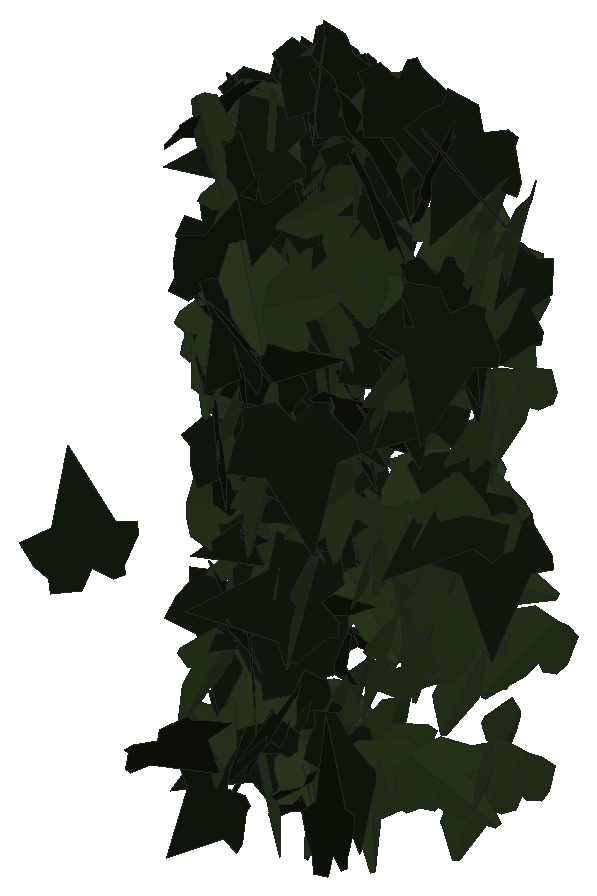
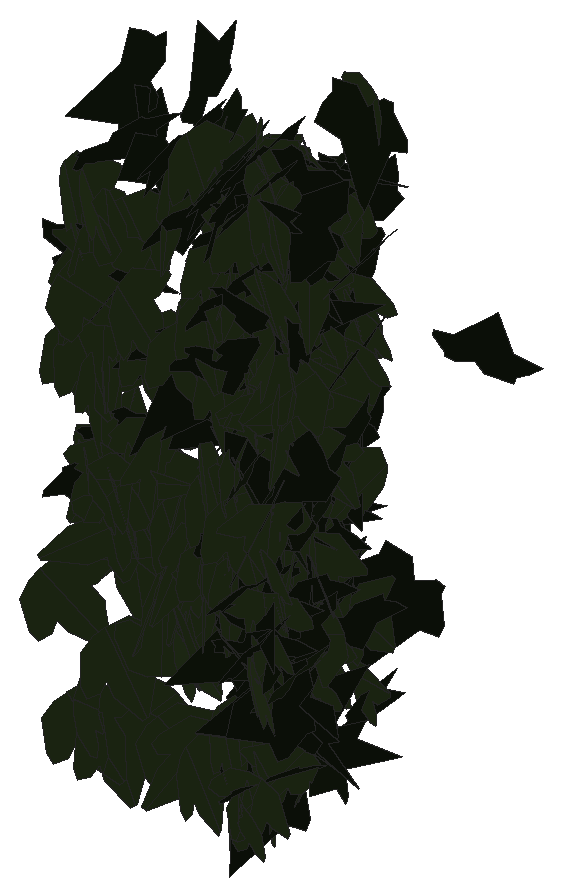
# SketchUp Ruby script. Lengths in inches.
U = 1.inch
M = Sketchup.active_model
def pt(a) = Geom::Point3d.new(a.map { |v| v * U })
def face(e, loops, mat)
  f = e.add_face(loops[0].map { |a| pt(a) })
  loops[1..].each { |l| e.add_face(l.map { |a| pt(a) }).erase! }
  f.material = f.back_material = mat if mat
  f
end
# faces: each face lists its corners as indices into pts; further lists are holes
def faces(e, pts, list, mat = nil) = list.each { |f| face(e, (f[0].is_a?(Array) ? f : [f]).map { |l| l.map { |i| pts[i] } }, mat) }
# xy, xz, yz: faces in a plane at the given z, y or x. An outline is a flat list of corners, or four numbers for a rectangle; further outlines are holes
def ring(l) = l.size == 4 ? [[l[0], l[1]], [l[2], l[1]], [l[2], l[3]], [l[0], l[3]]] : l.each_slice(2).to_a
def flat(e, list, mat, &to3) = list.each { |f| face(e, (f[0].is_a?(Array) ? f : [f]).map { |l| ring(l).map { |u, v| to3.(u, v) } }, mat) }
def xy(e, z, list, mat = nil) = flat(e, list, mat) { |x, y| [x, y, z] }
def xz(e, y, list, mat = nil) = flat(e, list, mat) { |x, z| [x, y, z] }
def yz(e, x, list, mat = nil) = flat(e, list, mat) { |y, z| [x, y, z] }
def lines(e, pts, list) = list.each { |a, b| e.add_line(pt(pts[a]), pt(pts[b])) }
# prism: a flat outline (further loops are holes) pulled along v
def prism(e, loops, v, mat = nil)
  f = face(e, loops, mat); d = Geom::Vector3d.new(v.map { |x| x * U })
  f.pushpull(f.normal.samedirection?(d) ? d.length : -d.length)
end
def box(e, o, s, mat = nil) = prism(e, [[o, [o[0] + s[0], o[1], o[2]], [o[0] + s[0], o[1] + s[1], o[2]], [o[0], o[1] + s[1], o[2]]]], [0, 0, s[2]], mat)
def at(x, y, z, deg = 0) = Geom::Transformation.translation(pt([x, y, z])) * Geom::Transformation.rotation(ORIGIN, Z_AXIS, deg.degrees)
def axes(o, x, y, z) = Geom::Transformation.new([*x, 0, *y, 0, *z, 0, *pt(o).to_a, 1])
def part(name) = M.definitions.add(name)
# library, detail: a bought-in or finely detailed component or shape, given as its bounding box
def library(name, o, s) = part(name).tap { |d| box(d.entities, o, s) }
def detail(e, o, s) = box(e.add_group.entities, o, s)
def put(e, d, t, mat = nil) = e.add_instance(d, t).tap { |i| i.material = mat if mat }
def group(e, t, mat = nil) = e.add_group.tap { |g| g.transformation = t; g.material = mat if mat }.entities
root = M.entities
M.materials.add("efeu1").color = [18, 25, 13]
M.materials.add("efeu2").color = [43, 57, 29]
c1 = part("ivyleaf_9")
p = [[1.54,2.16,1.25],[1.36,2.04,1.19],[-0.21,0.99,0.68],[-0.71,1.11,0.82],[-0.85,0.86,0.67],[-0.8,0.17,0.21],
  [-0.9,-0.01,0.1],[-0.67,-0.16,-0.02],[-0.08,-0.08,-0.05],[-0.03,-0.6,-0.4],[0.65,-0.88,-0.66],[0.83,-0.6,-0.49],
  [1.29,-0.42,-0.43],[1.8125,-0.07,-0.26],[1.21,0.44,0.15]]
faces(c1.entities,p,[[0,1,2,3,4,5,6,7,8,9,10,11,12,13,14]],"efeu1")
c2 = part("ivyleaf_10")
p = [[0,0.5,-0.03],[-0.0625,2.02,-0.43],[-0.19,2.01,-0.46],[-0.54,1.05,-0.29],[-0.52,0.625,-0.18],[-0.83,0.76,-0.28],
  [-1.16,0.64,-0.33],[-1.15,0.33,-0.24],[-0.77,-0.39,0.02],[-0.3,-0.51,0.16],[0.04,-0.48,0.23],[-0.02,2.01,-0.4375],
  [-0.06,2.01,-0.43],[0.04,-0.49,0.23],[0.67,-0.49,0.14],[1.38,0.36,-0.2],[1.375,0.51,-0.24],[0.81,0.65,-0.19],
  [0.62,0.59,-0.15],[0.6,1.09,-0.28],[0.5,1.23,-0.31]]
faces(c2.entities,p,[[0,1,2,3,4,5,6,7,8,9,10],[11,12,0,13,14,15,16,17,18,19,20]],"efeu2")
put(root,c1,axes([9.03,220.3,218.375],[-0.46158,-0.0625,0.05363],[0.05614,0.00087,0.44916],[-0.06712,0.43049,0.00688]))
put(root,c1,axes([9.21,221.32,215.71],[0.26243,0.35078,0.08782],[0.05444,0.0678,-0.44379],[-0.38585,0.24815,-0.00288]))
put(root,c1,axes([10.73,221.81,220.03],[-0.17094,-0.39097,-0.26062],[0.10894,0.2368,-0.42668],[0.45707,-0.20266,0.00422]))
put(root,c2,axes([10.66,222.125,217.94],[0.22138,-0.35038,0.27968],[0.16796,-0.22438,-0.41405],[0.41567,0.27728,0.01836]))
put(root,c1,axes([9.42,222.5,220.57],[-0.01869,-0.3188,0.38473],[-0.022,-0.3841,-0.31935],[0.49917,-0.02886,0.00033]))
put(root,c1,axes([9.09,222.61,214.48],[-0.1098,-0.3044,0.30539],[-0.09865,-0.27908,-0.33376],[0.44601,-0.13666,0.00136]))
put(root,c1,axes([9.27,222.56,219.99],[0.00235,-0.06151,0.4962],[0.13344,-0.47813,-0.0599],[0.48186,0.1327,0.01417]))
put(root,c1,axes([9.27,222.16,220.86],[0.45081,-0.04213,-0.11954],[-0.12069,0.03558,-0.43565],[0.05398,0.43149,0.02425]))
put(root,c1,axes([9.29,222.26,219.22],[0.12737,-0.03029,-0.43432],[-0.44087,0.0882,-0.12654],[0.1006,0.42489,-0.0047]))
put(root,c1,axes([9.15,222.26,221.14],[-0.10416,-0.16282,0.40735],[0.33014,0.2518,0.18714],[-0.3176,0.31514,0.06094]))
put(root,c2,axes([8.84,222.77,216.06],[0.00663,-0.31537,0.31153],[0.07081,-0.29549,-0.32493],[0.46439,0.04956,0.0451]))
put(root,c1,axes([10.82,222.36,214.46],[-0.06273,-0.27844,0.41053],[0.07774,0.40317,0.28533],[-0.48992,0.09963,-0.00729]))
put(root,c2,axes([9.42,222.51,221.33],[0.44175,0.16313,0.16806],[0.15784,0.05773,-0.47091],[-0.17304,0.4691,-0.00049]))
put(root,c2,axes([8.8,222.65,222.96],[-0.32377,0.16998,-0.27605],[0.1788,-0.22681,-0.34552],[-0.28968,-0.32998,0.09528]))
put(root,c2,axes([10.25,222.21,221.23],[0.01562,0.06077,0.49605],[-0.03337,0.49531,-0.05963],[-0.49864,-0.03125,0.01953]))
put(root,c2,axes([9.02,222.65,220.375],[0.45313,-0.05167,-0.10668],[-0.10708,0.03316,-0.43914],[0.06261,0.43065,0.02102]))
put(root,c1,axes([10.97,222.97,222.5],[0.05275,-0.25294,0.42806],[0.15413,-0.40094,-0.25591],[0.47272,0.15896,0.03567]))
put(root,c2,axes([9.09,222.51,214.99],[0.17526,0.02482,0.41895],[-0.42422,0.10948,0.15755],[-0.10016,-0.42027,0.06579]))
put(root,c1,axes([9.23,222.875,216.45],[-0.01029,-0.00016,-0.45229],[0.44401,-0.14186,-0.00931],[-0.15316,-0.41122,0.00339]))
put(root,c2,axes([8.83,222.75,220.08],[0.42796,-0.16072,0.08303],[0.08118,-0.02709,-0.4447],[0.176,0.40331,0.00321]))
put(root,c2,axes([10.42,223.05,218.47],[-0.01229,0.03434,-0.49867],[-0.10712,-0.48741,-0.03093],[-0.48823,0.10608,0.01934]))
put(root,c1,axes([10.09,222.99,217.0625],[-0.2627,-0.11378,0.40993],[-0.38104,-0.15135,-0.28619],[0.18921,-0.46276,-0.00719]))
put(root,c1,axes([8.99,223.03,216.43],[-0.08964,-0.12573,0.4244],[0.09415,-0.41195,-0.11356],[0.45146,0.06094,0.10795]))
put(root,c2,axes([9.4,222.91,218.43],[0.08814,-0.41194,0.118],[0.0821,-0.09967,-0.43321],[0.4541,0.09798,0.05542]))
put(root,c1,axes([9.2,222.53,219.97],[0.12506,0.23578,-0.3606],[0.13456,0.32412,0.27249],[0.4324,-0.16906,0.0195]))
put(root,c1,axes([9.0625,222.77,219.0625],[-0.02483,-0.21345,-0.39347],[0.04001,0.37652,-0.22326],[0.46743,-0.04357,-0.00179]))
put(root,c2,axes([9.36,223.04,217.41],[0.37611,-0.26062,-0.00539],[-0.00274,0.00527,-0.45236],[0.28151,0.34825,0.00281]))
put(root,c1,axes([9.11,223.34,222],[-0.04348,-0.42405,0.26132],[0.09475,-0.26456,-0.41356],[0.48901,0.01356,0.10336]))
put(root,c1,axes([8.73,222.75,222.94],[0.03171,0.4311,0.05217],[-0.01873,0.05141,-0.44887],[-0.46835,0.02713,0.02148]))
put(root,c2,axes([9.16,222.64,218.96],[0.00573,-0.01075,0.49985],[-0.23319,0.44213,0.01219],[-0.44226,-0.23326,0.00006]))
put(root,c1,axes([10.01,222.84,216.32],[-0.49514,0.06082,-0.03374],[-0.03471,-0.00594,0.49876],[0.06027,0.49625,0.0101]))
put(root,c2,axes([8.7,222.71,217.95],[-0.02151,0.13732,0.42877],[-0.09106,0.40364,-0.14406],[-0.46039,-0.08625,0.00847]))
put(root,c2,axes([9.44,223.07,217.58],[-0.4481,-0.0202,-0.13429],[0.14111,-0.07352,-0.42468],[-0.00309,-0.42827,0.07924]))
put(root,c1,axes([9.14,223.08,218.62],[0.05465,0.32878,-0.29151],[-0.03152,-0.27897,-0.34579],[-0.46555,0.05748,-0.01081]))
put(root,c2,axes([8.83,223.32,221.77],[-0.02166,-0.43323,0.24869],[0.08934,-0.24827,-0.42471],[0.49148,0.02604,0.08817]))
put(root,c2,axes([8.875,222.91,219.44],[-0.06862,-0.29912,0.32175],[0.14762,0.28251,0.31326],[-0.44069,0.14121,0.05483]))
put(root,c2,axes([10.69,223.12,221.6],[-0.28981,-0.40644,-0.02856],[0.02022,0.02066,-0.49916],[0.40694,-0.29048,0.00446]))
put(root,c2,axes([10.11,223.5,221.98],[-0.03684,0.00806,-0.49858],[-0.19231,-0.46149,0.00674],[-0.46007,0.19225,0.0371]))
put(root,c2,axes([8.62,223.2,219.91],[0.46238,-0.05871,0.05184],[0.05266,-0.01132,-0.44939],[0.06438,0.43087,-0.00474]))
put(root,c1,axes([8.54,223.15,219.91],[0.24209,-0.34244,-0.15325],[-0.08637,0.12377,-0.42565],[0.39325,0.238,0.00085]))
put(root,c2,axes([9.22,223.2,215.76],[0.42562,-0.03527,-0.18798],[-0.19329,0.02724,-0.41136],[0.04686,0.43271,0.01057]))
put(root,c1,axes([8.43,223.1,221.23],[0.28955,-0.26425,-0.22671],[-0.07049,0.23234,-0.37639],[0.36319,0.25577,0.10769]))
put(root,c1,axes([8.54,223.4,216.39],[-0.12336,-0.41727,-0.04726],[0.00804,0.04508,-0.4499],[0.45324,-0.11437,-0.00488]))
put(root,c2,axes([9.32,223.28,216.97],[0.32785,-0.31085,0.02205],[0.02187,-0.00986,-0.45179],[0.33578,0.30414,0.0079]))
put(root,c1,axes([9.43,223.08,217.51],[0.35392,0.22866,-0.17878],[-0.15606,-0.0933,-0.41553],[-0.26665,0.3581,0.0059]))
put(root,c2,axes([8.92,223.4,217.03],[-0.08977,-0.40031,0.1545],[0.00536,-0.15224,-0.42376],[0.46111,-0.07616,0.035]))
put(root,c2,axes([8.91,223.3,221.82],[0.10653,0.41027,-0.10992],[-0.01722,-0.10485,-0.43875],[-0.45724,0.09953,-0.00909]))
put(root,c1,axes([11.57,223.48,220.98],[-0.2158,-0.44692,-0.06078],[0.01984,0.05791,-0.49624],[0.4506,-0.21659,-0.00726]))
put(root,c1,axes([9.67,223.57,217.65],[-0.07482,-0.16229,-0.46697],[-0.14702,-0.44362,0.17773],[-0.47201,0.1639,0.01866]))
put(root,c1,axes([9.54,223.28,215.67],[-0.36534,0.31347,-0.13513],[0.09923,-0.09185,-0.48137],[-0.32661,-0.37855,0.0049]))
put(root,c1,axes([9.23,223.46,222.31],[-0.40457,0.03361,0.2273],[-0.23271,-0.15205,-0.35978],[0.05364,-0.40617,0.15349]))
put(root,c1,axes([9.14,223.4375,217.45],[-0.36975,-0.23851,-0.12791],[0.11366,0.06406,-0.43387],[0.2666,-0.3581,0.00758]))
put(root,c1,axes([8.45,223.53,218.86],[0.1033,-0.26844,0.34181],[0.17592,-0.28787,-0.29383],[0.42319,0.18519,0.03871]))
put(root,c1,axes([9.27,223.39,215.43],[-0.41423,0.11986,-0.17325],[0.16997,-0.05485,-0.41788],[-0.14225,-0.41455,0.0052]))
put(root,c2,axes([8.99,222.97,218.56],[0.09536,0.07108,-0.43677],[0.12435,0.40895,0.09716],[0.44289,-0.13012,0.06676]))
put(root,c2,axes([9.3,223.3,216.5],[-0.46868,0.02099,-0.0224],[0.02338,0.00172,-0.45184],[-0.02255,-0.43449,-0.00287]))
put(root,c2,axes([9.38,223.46,216.63],[0.01987,-0.06414,0.44705],[0.4645,-0.05918,-0.02833],[0.06749,0.42616,0.06335]))
put(root,c2,axes([9.03,223.4,214.33],[-0.19082,0.3726,-0.14402],[0.07838,-0.11876,-0.42862],[-0.42209,-0.1905,-0.01448]))
put(root,c1,axes([8.88,223.75,216.34],[-0.15985,-0.25869,0.32953],[-0.10036,-0.30689,-0.30571],[0.43022,-0.16771,0.05112]))
put(root,c1,axes([8.79,223.74,214.58],[-0.2676,-0.24176,0.27394],[-0.2073,-0.18043,-0.36001],[0.32578,-0.3134,-0.00406]))
put(root,c1,axes([9.28,223.13,216.61],[0.01529,0.19307,-0.40513],[0.03438,0.38825,0.20133],[0.46829,-0.03481,-0.00155]))
put(root,c2,axes([9.08,223.61,220.64],[0.31984,-0.07259,0.3774],[0.36817,-0.08293,-0.32798],[0.11022,0.4877,0.0004]))
put(root,c2,axes([8.49,223.29,219.35],[-0.11056,-0.17572,0.39992],[0.18022,0.34673,0.21099],[-0.41954,0.19525,-0.01475]))
put(root,c1,axes([8.65,223.57,218.0625],[0.29197,-0.33536,-0.06304],[-0.04528,0.04406,-0.44796],[0.36526,0.27353,-0.00514]))
put(root,c1,axes([9.51,223.74,220.19],[-0.20361,-0.01355,0.45646],[-0.44659,-0.09849,-0.20213],[0.09539,-0.49002,0.028]))
put(root,c1,axes([8.9375,223.19,214.41],[0.01325,0.24649,0.37254],[-0.01602,0.35838,-0.25595],[-0.46934,-0.00527,0.01925]))
put(root,c2,axes([9.9375,223.45,218.46],[0.23032,-0.16029,-0.41384],[-0.35062,0.22011,-0.28039],[0.27207,0.41935,-0.01101]))
put(root,c2,axes([8.88,223.61,218.6875],[0.38806,0.0951,-0.23503],[-0.24366,-0.02874,-0.38564],[-0.10368,0.4235,0.02661]))
put(root,c2,axes([9.23,223.58,216.37],[-0.01532,-0.43142,-0.05603],[0.00706,0.05369,-0.44889],[0.4695,-0.01489,0.00492]))
put(root,c2,axes([9.73,223.58,220.39],[-0.41132,0.22303,-0.17629],[0.14968,-0.09369,-0.46778],[-0.24169,-0.43758,0.0103]))
put(root,c2,axes([8.75,223.7,222.58],[0.41901,-0.26337,0.07117],[0.05547,-0.04547,-0.49483],[0.26712,0.42257,-0.00889]))
put(root,c2,axes([10.63,223.75,219.85],[0.14575,-0.46449,0.11403],[0.02634,-0.11123,-0.48676],[0.47756,0.1479,-0.00795]))
put(root,c2,axes([9.05,223.87,219.4],[0.06841,-0.40047,0.29146],[0.10932,-0.27476,-0.40318],[0.48308,0.11888,0.04997]))
put(root,c1,axes([9.06,223.97,219.75],[0.03379,-0.4078,0.28732],[0.01885,-0.28673,-0.40918],[0.4985,0.03849,-0.004]))
put(root,c1,axes([9.15,223.8,214.8],[0.07908,0.02221,0.44535],[-0.45198,-0.0909,0.07933],[0.10085,-0.42482,0.00631]))
put(root,c1,axes([8.81,223.8,216.78],[-0.08652,0.15145,0.41583],[0.07176,-0.39744,0.17041],[0.45615,0.09125,0.05207]))
put(root,c2,axes([8.58,223.88,217.32],[0.27744,-0.24845,0.33362],[0.24991,-0.22102,-0.37242],[0.33253,0.37339,0.00154]))
put(root,c1,axes([9.85,223.87,214.84],[0.06478,-0.42949,0.03555],[0.00215,-0.03424,-0.45099],[0.46531,0.05995,-0.00286]))
put(root,c1,axes([9.19,223.86,221.27],[-0.44915,-0.11934,-0.04682],[0.0454,0.0167,-0.44995],[0.13006,-0.41798,-0.00461]))
put(root,c1,axes([11.29,223.74,222.86],[0.4191,-0.2436,0.12255],[0.10726,-0.05932,-0.48474],[0.25071,0.4326,0.00254]))
put(root,c2,axes([8.92,223.54,218.86],[-0.24255,0.27409,0.26241],[-0.20391,0.17023,-0.3671],[-0.34684,-0.29176,0.03231]))
put(root,c1,axes([9.15,223.78,219.9],[0.09149,-0.39072,-0.17827],[-0.03012,0.16932,-0.41571],[0.45982,0.08884,0.00824]))
put(root,c2,axes([9.05,223.85,219.64],[-0.33047,-0.26849,0.15946],[-0.07125,-0.15405,-0.41748],[0.32623,-0.30562,0.07035]))
put(root,c1,axes([11.11,223.89,221.12],[0.18721,-0.45701,-0.07806],[-0.02016,0.07608,-0.49377],[0.46319,0.18803,0.01006]))
put(root,c2,axes([9.17,223.72,220.75],[-0.11235,0.42121,0.03269],[-0.05251,0.02022,-0.44907],[-0.45314,-0.10678,0.04394]))
put(root,c2,axes([8.47,223.84,216.39],[-0.18964,0.05491,-0.40995],[0.40267,-0.12801,-0.19128],[-0.15035,-0.4121,0.0048]))
put(root,c2,axes([8.72,223.79,217.39],[-0.37313,-0.26418,0.00853],[-0.00552,-0.00682,-0.45231],[0.2854,-0.34552,0.0024]))
put(root,c2,axes([9.21,224.09,217.49],[0.09817,-0.15207,0.46609],[0.3736,-0.28459,-0.17154],[0.31746,0.38195,0.05775]))
put(root,c2,axes([9.33,223.8,214.4],[0.37527,0.12635,0.23835],[0.23553,0.07077,-0.38445],[-0.15623,0.41018,-0.00709]))
put(root,c2,axes([9.2,223.9375,214.23],[-0.25074,0.24324,-0.28701],[0.17486,-0.22546,-0.34833],[-0.35674,-0.28147,0.03099]))
put(root,c2,axes([9.49,224.08,219.88],[0.1972,-0.28926,0.35699],[0.29023,-0.22276,-0.34081],[0.35621,0.34163,0.08005]))
put(root,c1,axes([9.6875,223.66,219.05],[0.42875,0.08447,0.16274],[0.16067,0.05192,-0.42168],[-0.10521,0.42355,0.01924]))
put(root,c2,axes([9.84,224.125,222.35],[0.19986,-0.23907,0.39102],[0.28612,-0.26816,-0.3102],[0.35804,0.34775,0.02961]))
put(root,c2,axes([9.38,223.96,214.1],[0.37294,-0.25718,0.06449],[0.05815,-0.0315,-0.44772],[0.27973,0.34942,0.0071]))
put(root,c2,axes([8.9375,223.79,215.52],[-0.17137,-0.37597,-0.15668],[0.05609,0.14158,-0.42434],[0.43382,-0.16682,-0.00703]))
put(root,c2,axes([9.18,223.82,220.77],[-0.42187,0.13162,0.14455],[-0.15215,0.01619,-0.42769],[-0.13997,-0.41429,0.02921]))
put(root,c1,axes([9.93,224.11,222.57],[0.23236,-0.38986,0.2098],[0.12115,-0.17191,-0.45362],[0.42583,0.26164,0.01457]))
put(root,c2,axes([11.01,224.19,218.09],[0.03789,-0.37967,0.32314],[0.09056,-0.31344,-0.37889],[0.49027,0.08724,0.04501]))
put(root,c1,axes([8.6,224.17,215.85],[0.06508,-0.40376,0.15624],[0.03414,-0.14714,-0.42446],[0.46402,0.06746,0.00932]))
put(root,c2,axes([8.5,223.87,222.25],[-0.17844,-0.08088,-0.40995],[0.43164,0.01657,-0.17776],[0.05054,-0.42709,0.07074]))
put(root,c1,axes([9.33,223.82,219.23],[0.30334,-0.26881,-0.20295],[-0.0503,0.22116,-0.38655],[0.3552,0.26088,0.11857]))
put(root,c1,axes([9.27,224.12,219.55],[0.24832,-0.33868,0.27135],[0.18063,-0.2036,-0.41943],[0.3946,0.30633,0.02124]))
put(root,c1,axes([10.83,224.3,219.58],[-0.32357,-0.30409,0.22985],[-0.12649,-0.19876,-0.44102],[0.35959,-0.34354,0.05169]))
put(root,c2,axes([9.91,224.08,214.26],[0.37841,-0.14662,0.29207],[0.27407,-0.10103,-0.4058],[0.17802,0.46722,0.00391]))
put(root,c1,axes([8.875,224.07,215.27],[-0.46831,-0.00338,-0.03586],[0.03721,0.00291,-0.45097],[0.00389,-0.43498,-0.00274]))
put(root,c2,axes([8.375,223.8125,222.35],[0.21963,0.15528,0.36586],[0.31426,0.19802,-0.26584],[-0.2715,0.35482,-0.01174]))
put(root,c2,axes([8.63,223.93,221.35],[-0.02185,-0.48705,-0.11093],[0.02128,0.11003,-0.48728],[0.49907,-0.02602,0.01592]))
put(root,c1,axes([10.01,224.05,222.18],[0.04922,-0.45909,-0.19187],[0.03354,0.19543,-0.459],[0.49644,0.03231,0.05003]))
put(root,c2,axes([8.9,223.97,219.56],[0.31547,0.32225,0.0076],[0.00511,0.00558,-0.45234],[-0.34809,0.29214,0.00025]))
put(root,c1,axes([8.48,224,216.58],[0.38475,-0.19246,0.16532],[0.15287,-0.07243,-0.4211],[0.22206,0.38332,0.00344]))
put(root,c1,axes([8.73,224.19,216.99],[-0.22055,-0.38232,-0.03833],[0.01642,0.03366,-0.45077],[0.41449,-0.20476,-0.00254]))
put(root,c1,axes([11.41,224.26,218.34],[-0.42607,-0.23159,0.1218],[-0.10502,-0.06184,-0.48492],[0.23967,-0.4388,0.00405]))
put(root,c1,axes([9.71,224.11,217.78],[-0.378,0.03105,0.26669],[-0.27774,-0.0014,-0.36487],[-0.02616,-0.43389,0.02026]))
put(root,c2,axes([10.91,224.1,219.65],[-0.15467,-0.47063,0.06774],[-0.01512,-0.06633,-0.49535],[0.47524,-0.15528,0.00629]))
put(root,c2,axes([9.64,224.05,218.3],[-0.265,-0.35776,0.03328],[-0.01947,-0.02643,-0.45117],[0.38743,-0.24604,0.00008]))
put(root,c1,axes([10.37,224.17,219.99],[-0.0592,-0.47163,-0.15511],[0.0552,0.14899,-0.47408],[0.49341,-0.07325,0.03442]))
put(root,c2,axes([11.41,224.17,217.78],[-0.40967,-0.2596,-0.12157],[-0.10417,-0.06273,0.48499],[-0.26706,0.4227,-0.00269]))
put(root,c2,axes([8.57,224.37,220.63],[-0.0336,-0.10346,-0.43823],[0.01702,-0.42244,0.10666],[-0.46829,-0.00793,0.03532]))
put(root,c1,axes([9.3125,223.78,214.09],[0.22095,0.3772,0.07417],[0.03618,0.06297,-0.44628],[-0.41302,0.20731,0.00059]))
put(root,c2,axes([9.46,224,219.42],[-0.10954,0.42293,0.00848],[-0.00026,0.00833,-0.45232],[-0.45685,-0.10141,-0.00177]))
put(root,c2,axes([9.7,224.03,217.73],[-0.45809,0.0909,-0.03375],[0.03397,-0.00807,-0.45114],[-0.09855,-0.42532,0.00134]))
put(root,c2,axes([9.45,224.18,217.75],[0.31963,-0.31673,0.03783],[0.02611,-0.0272,-0.45081],[0.34332,0.29694,-0.00094]))
put(root,c2,axes([9.21,224.41,218.65],[0.03901,-0.30822,0.39176],[0.20334,-0.34894,-0.29478],[0.45512,0.18232,0.09812]))
put(root,c1,axes([8.51,224.29,220.41],[0.02135,0.17757,0.41248],[-0.06081,-0.39263,0.18573],[0.46536,-0.05945,0.00535]))
put(root,c2,axes([11.26,224.11,216.8],[-0.45801,-0.13356,0.14963],[-0.13872,-0.05845,-0.4768],[0.14485,-0.47828,0.01648]))
put(root,c2,axes([10.47,224.29,214.52],[-0.27954,-0.2476,0.3325],[-0.2162,-0.25511,-0.37172],[0.35372,-0.35159,0.03556]))
put(root,c1,axes([8.74,224.36,217.72],[0.05568,-0.25111,0.42877],[0.29824,-0.3282,-0.23095],[0.39743,0.28147,0.11323]))
put(root,c1,axes([8.98,224.31,215.55],[-0.07293,-0.12433,0.4278],[0.31206,-0.32135,-0.05168],[0.34353,0.26552,0.13777]))
put(root,c1,axes([11.06,224.37,220.6],[0.12857,-0.47212,0.10284],[0.02435,-0.09995,-0.4893],[0.48257,0.13083,-0.00271]))
put(root,c2,axes([9.19,224.18,214.99],[-0.30175,-0.31725,0.10665],[-0.07976,-0.07159,-0.43957],[0.35114,-0.28888,-0.00819]))
put(root,c2,axes([10.82,224.15,218.47],[0.36422,0.34168,-0.02438],[-0.01894,-0.01544,-0.4994],[-0.34203,0.36471,0.0017]))
put(root,c2,axes([8.68,224.42,222.19],[0.11257,-0.35837,0.33],[0.1567,-0.29406,-0.37279],[0.46127,0.18735,0.04611]))
put(root,c2,axes([11.02,224.35,217.35],[0.03216,-0.45689,0.20055],[0.03512,-0.19839,-0.45761],[0.49773,0.04352,0.01933]))
put(root,c1,axes([8.6,224.09,222.72],[-0.04813,-0.19628,-0.45734],[0.26816,0.37684,-0.18996],[0.41925,-0.26357,0.06899]))
put(root,c2,axes([8.83,224.37,215.24],[-0.01047,-0.45858,0.19899],[0.02192,-0.19927,-0.45805],[0.49941,-0.00087,0.02427]))
put(root,c2,axes([9.54,224.5,217.32],[-0.0452,-0.3396,0.36418],[0.03221,-0.36691,-0.33814],[0.49691,-0.00711,0.05505]))
put(root,c2,axes([8.58,224.43,219.96],[-0.03407,0.07255,-0.44486],[0.24707,-0.36163,-0.08134],[-0.39813,-0.23062,-0.0124]))
put(root,c2,axes([10.58,224.33,217.93],[-0.20614,-0.42845,0.15471],[-0.06078,-0.14242,-0.47542],[0.45146,-0.21481,0.00663]))
put(root,c2,axes([10.8,224.11,214.71],[-0.32667,-0.13011,-0.35547],[0.34508,0.09061,-0.3503],[0.15557,-0.4742,0.0306]))
put(root,c1,axes([8.48,224.03,222.01],[0.42703,0.08004,0.16923],[0.17173,0.03459,-0.41955],[-0.09414,0.42617,0.00227]))
put(root,c1,axes([8.21,224.22,222.18],[0.37852,-0.16525,0.28181],[0.26665,-0.0929,-0.41263],[0.18873,0.46267,0.01779]))
put(root,c1,axes([11.52,224.41,217.85],[-0.13765,-0.46733,-0.11251],[0.03708,0.10636,-0.48715],[0.47925,-0.14245,0.00537]))
put(root,c1,axes([10.97,223.82,222.22],[0.02245,0.21261,0.45199],[0.07401,0.44603,-0.21349],[-0.49398,0.07649,-0.01144]))
put(root,c2,axes([11.01,224.3,217.04],[-0.36525,-0.34061,0.02407],[0.02269,0.01095,0.49936],[-0.3407,0.36588,0.00746]))
put(root,c2,axes([10.04,224.5,215.99],[0.13553,-0.41583,0.24231],[0.06296,-0.23426,-0.43722],[0.47714,0.14903,-0.01114]))
put(root,c1,axes([9.3,224.21,218.43],[-0.33459,0.30526,0.00802],[-0.00407,0.00716,-0.45232],[-0.32976,-0.30982,-0.00255]))
put(root,c1,axes([10.02,224.07,219.57],[0.48761,0.11054,0.00464],[0.0041,0.00289,-0.49997],[-0.11056,0.48762,0.00191]))
put(root,c2,axes([8.95,224.45,222.93],[0.27319,-0.24045,0.27005],[0.21788,-0.16426,-0.36258],[0.31402,0.32315,0.01663]))
put(root,c2,axes([9.1875,224.22,217.8],[-0.35197,0.28607,-0.03563],[0.03515,-0.01485,-0.45087],[-0.30918,-0.32736,-0.01069]))
put(root,c2,axes([8.91,224.14,218.03],[0.18574,-0.37804,-0.26941],[-0.05279,0.27109,-0.4168],[0.46121,0.18328,0.06079]))
put(root,c2,axes([10.75,224.01,216.4],[0.13696,-0.2891,-0.38427],[0.04146,0.40516,-0.29004],[0.47908,0.04758,0.13496]))
put(root,c2,axes([9.3,224.43,218.66],[0.00826,-0.48529,0.12009],[0.02597,-0.11953,-0.48481],[0.49926,0.01425,0.02323]))
put(root,c2,axes([10.52,224.44,215.67],[-0.21832,-0.43728,-0.10546],[-0.02816,-0.10371,0.48832],[-0.44894,0.21915,0.02066]))
put(root,c2,axes([9.07,224.51,216.17],[0.17833,-0.25636,0.32263],[0.24465,-0.21794,-0.31271],[0.35924,0.27569,0.05281]))
put(root,c2,axes([9.68,224.22,216.53],[0.3428,0.1539,0.26472],[0.23382,0.13573,-0.36612],[-0.22028,0.38356,0.02334]))
put(root,c2,axes([10.26,224.22,216.8],[-0.42605,0.2616,-0.00675],[0.0101,0.00355,-0.49989],[-0.26149,-0.42609,-0.00831]))
put(root,c2,axes([8.88,224.4375,216.64],[0.08243,-0.48425,0.0933],[0.03515,-0.08859,-0.49083],[0.49191,0.08747,0.01943]))
put(root,c2,axes([8.73,224.19,219.6],[-0.1618,-0.10636,-0.46099],[0.4532,0.10497,-0.18328],[0.13577,-0.47715,0.06244]))
put(root,c1,axes([8.46,224.48,216.11],[0.1686,-0.38667,0.1288],[0.14598,-0.07562,-0.42275],[0.41349,0.18436,0.09673]))
put(root,c2,axes([8.9,224.52,222.85],[0.03258,-0.3834,0.2114],[0.01362,-0.2029,-0.39996],[0.46847,0.03257,-0.00307]))
put(root,c2,axes([10.9375,224.49,221.47],[-0.30357,-0.33775,0.20921],[-0.065,-0.21752,-0.44549],[0.39194,-0.29767,0.08816]))
put(root,c1,axes([8.97,224.34,218.49],[0.35501,-0.27963,-0.05675],[-0.0427,0.03773,-0.44882],[0.30472,0.33107,0.00322]))
put(root,c2,axes([9.02,224.41,218.98],[0.49193,-0.03411,0.08272],[0.08265,-0.00384,-0.49311],[0.03427,0.49882,0.00186]))
put(root,c2,axes([9.61,224.38,219.74],[-0.08179,-0.49228,-0.03109],[0.00625,0.03048,-0.49903],[0.49322,-0.08202,0.00117]))
put(root,c1,axes([8.7,223.96,215.49],[-0.01088,0.26345,-0.42483],[-0.00459,0.42486,0.26358],[0.49986,0.00963,-0.00683]))
put(root,c2,axes([8.9,224.27,216.86],[-0.28857,0.34232,0.02651],[-0.0093,0.02561,-0.45153],[-0.37061,-0.26719,-0.00932]))
put(root,c2,axes([10.47,224.23,217.55],[-0.31012,0.37538,0.11365],[-0.08692,0.07551,-0.48656],[-0.38245,-0.32154,0.01842]))
put(root,c1,axes([8.96,224.36,223.03],[0.21048,-0.40356,-0.20698],[-0.05481,0.20388,-0.45324],[0.45022,0.21348,0.04159]))
put(root,c2,axes([11.53,224.25,219.6875],[0.3121,-0.31093,-0.23646],[-0.07492,0.2494,-0.42683],[0.38338,0.30186,0.10909]))
put(root,c2,axes([9.375,224.3,222.11],[0.02294,-0.47271,-0.1613],[0.0337,0.16257,-0.47163],[0.49834,0.01077,0.03932]))
put(root,c1,axes([11.04,224.72,222.57],[-0.2029,-0.43954,0.12507],[-0.00293,-0.13558,-0.48126],[0.45697,-0.19602,0.05244]))
put(root,c2,axes([11.39,224.51,221.27],[-0.00666,0.44172,-0.23417],[-0.08551,-0.23175,-0.43472],[-0.49259,0.03426,0.07863]))
put(root,c1,axes([9.06,224.52,218.81],[0.24925,-0.3628,0.06854],[0.04221,-0.05324,-0.44716],[0.39599,0.23403,0.00453]))
put(root,c1,axes([8.92,224.74,222.48],[-0.05091,-0.45172,0.20823],[0.00524,-0.20979,-0.45383],[0.49737,-0.04403,0.02609]))
put(root,c1,axes([9.93,224.62,222],[0.01287,-0.49848,-0.03676],[-0.00195,0.03673,-0.49865],[0.49983,0.01298,-0.001]))
put(root,c1,axes([8.4375,224.41,218.52],[0.0684,-0.10484,0.4341],[0.44876,-0.09495,-0.09037],[0.12102,0.41136,0.08977]))
put(root,c1,axes([9.3,224.75,222.04],[-0.13662,-0.46684,0.11574],[-0.02972,-0.1119,-0.48641],[0.48005,-0.13979,0.00283]))
put(root,c1,axes([8.76,224.71,214.64],[-0.16,-0.40649,0.04698],[0.09094,-0.07733,-0.4365],[0.43225,-0.1342,0.10922]))
put(root,c1,axes([9.26,224.68,217.84],[-0.30257,-0.33244,0.0154],[-0.00411,-0.01615,-0.45207],[0.35937,-0.28009,0.00779]))
put(root,c2,axes([9.6,224.52,217.33],[-0.34484,-0.3277,0.15394],[-0.09226,-0.12604,-0.47498],[0.35011,-0.35599,0.02646]))
put(root,c1,axes([8.9375,224.66,216.93],[-0.33824,-0.30167,-0.01216],[0.00754,0.00961,-0.45223],[0.32596,-0.31326,-0.00216]))
put(root,c2,axes([10.15,224.53,216.37],[0.35694,-0.35009,0.00527],[0.00397,-0.00347,-0.49997],[0.35011,0.35696,0.00031]))
put(root,c2,axes([10.03,224.25,214.53],[-0.22174,-0.284,-0.34667],[0.23734,0.25366,-0.35962],[0.38013,-0.32404,0.02231]))
put(root,c2,axes([11.17,224.58,214.4375],[-0.24432,-0.41028,0.14824],[-0.03654,-0.15007,-0.47555],[0.43471,-0.2432,0.04335]))
put(root,c2,axes([8.6875,224.33,217.51],[-0.32743,0.29118,0.11639],[-0.09356,0.07132,-0.43709],[-0.32365,-0.3152,0.00861]))
put(root,c2,axes([11.4,224.45,219.2],[-0.03318,-0.49214,-0.08186],[0.01717,0.08087,-0.49312],[0.4986,-0.03554,0.01153]))
put(root,c1,axes([9.1,224.67,222.32],[-0.44582,-0.10843,0.08744],[-0.07899,-0.05163,-0.44272],[0.12537,-0.41809,0.03199]))
put(root,c2,axes([10.22,224.61,217.63],[0.02471,-0.49107,0.09078],[0.01583,-0.09007,-0.49157],[0.49914,0.02717,0.01109]))
put(root,c1,axes([10.03,224.56,222.94],[0.16527,-0.45327,-0.13126],[-0.01634,0.1335,-0.48157],[0.47161,0.16346,0.02932]))
put(root,c2,axes([8.44,224.41,220.0625],[-0.34061,-0.05216,-0.30683],[0.31376,0.05144,-0.33244],[0.07907,-0.42879,-0.00256]))
put(root,c2,axes([9,224.625,222.04],[-0.28234,-0.39865,0.10659],[0.02038,-0.14247,-0.47884],[0.41215,-0.26605,0.0967]))
put(root,c2,axes([9.85,224.64,222.79],[-0.05678,-0.48268,0.11744],[0.01305,-0.11962,-0.48531],[0.49659,-0.05204,0.02619]))
put(root,c2,axes([11.52,224.65,219.6],[-0.13176,-0.46015,0.14457],[-0.03887,-0.13925,-0.47864],[0.48076,-0.13737,0.00092]))
put(root,c2,axes([9.3,224.36,221.16],[-0.08606,-0.41834,-0.25998],[0.09164,0.24571,-0.42571],[0.48394,-0.12092,0.03438]))
put(root,c1,axes([11.8,224.57,220.72],[-0.34124,0.06496,0.35963],[-0.35124,0.07757,-0.34729],[-0.10091,-0.48966,-0.00731]))
put(root,c1,axes([9.21,224.78,222.87],[0.04461,-0.39332,0.1884],[0.06263,-0.17531,-0.40962],[0.46346,0.06155,0.03722]))
put(root,c2,axes([11.61,224.38,220.58],[-0.17486,-0.40548,-0.23455],[0.09535,0.21431,-0.44157],[0.45862,-0.19915,0.00238]))
put(root,c2,axes([9.81,224.38,217.07],[0.12813,-0.40307,-0.26668],[-0.04329,0.26522,-0.42165],[0.48136,0.13114,0.03307]))
put(root,c2,axes([8.81,224.58,216.59],[0.40647,-0.21811,0.00313],[0.00807,0.00689,-0.45228],[0.23544,0.37631,0.01009]))
put(root,c2,axes([8.73,224.3125,219.58],[0.06971,-0.34291,-0.35714],[-0.05513,0.35305,-0.34974],[0.49204,0.08814,0.01141]))
put(root,c2,axes([11.62,224.62,219.65],[-0.24214,-0.42719,0.0942],[-0.03615,-0.08775,-0.49091],[0.43596,-0.24455,0.01161]))
put(root,c1,axes([9.3,224.58,222.71],[0.18873,-0.43646,-0.15454],[-0.04306,0.14962,-0.47514],[0.46101,0.19266,0.01889]))
put(root,c1,axes([9.19,224.38,217.4],[0.15165,0.11795,-0.46162],[-0.46887,-0.04914,-0.16658],[-0.08467,0.4834,0.0957]))
put(root,c2,axes([9.36,224.49,217.12],[-0.05373,-0.40902,-0.14504],[0.01226,0.1391,-0.42848],[0.46656,-0.05076,-0.00545]))
put(root,c1,axes([8.9375,224.77,216.49],[-0.36622,-0.27218,-0.01323],[0.01197,0.00651,-0.4522],[0.29403,-0.33927,0.00194]))
put(root,c2,axes([9.94,224.73,220.23],[-0.28299,-0.37863,0.16295],[0.01742,-0.20847,-0.45414],[0.41184,-0.25136,0.13118]))
put(root,c2,axes([9.63,224.68,218.22],[0.01978,-0.49363,0.07706],[0.00013,-0.07711,-0.49402],[0.49961,0.01956,-0.00292]))
put(root,c2,axes([9.375,224.625,215.16],[0.08523,-0.49255,-0.0115],[0.00005,0.01168,-0.49986],[0.49268,0.08521,0.00204]))
put(root,c1,axes([8.86,224.6875,217.29],[0.05261,-0.42142,-0.10006],[0.06047,0.10216,-0.43588],[0.46291,0.03455,0.06831]))
put(root,c1,axes([9.27,224.66,216.33],[-0.43158,0.16022,-0.06464],[0.05167,-0.04739,-0.44695],[-0.17827,-0.40163,0.02695]))
put(root,c2,axes([8.7,224.68,217.64],[0.36984,-0.26816,0.00726],[0.00582,-0.00445,-0.45234],[0.28965,0.34248,-0.00018]))
put(root,c2,axes([8.72,224.67,221.4],[0.42935,-0.17495,-0.02493],[-0.02275,0.01164,-0.45171],[0.18935,0.3981,0.00225]))
put(root,c2,axes([11.22,224.96,214.96],[0.10835,-0.2672,0.40849],[0.18288,-0.36573,-0.28774],[0.45256,0.21176,0.01848]))
put(root,c2,axes([11.26,224.78,217.9],[0.37281,-0.2048,0.2628],[0.24358,-0.10156,-0.42468],[0.22733,0.44468,0.02405]))
put(root,c2,axes([8.69,224.73,222.53],[0.08474,-0.49127,0.03841],[0.00131,-0.03875,-0.49849],[0.49276,0.08459,-0.00528]))
put(root,c1,axes([9.19,224.87,221.21],[-0.0506,-0.43099,0.03713],[-0.01132,-0.03477,-0.45082],[0.46693,-0.04755,-0.0069]))
put(root,c2,axes([8.53,224.44,214.89],[0.15441,0.29901,0.29301],[0.13759,0.25134,-0.34465],[-0.42183,0.19143,-0.00516]))
put(root,c2,axes([11.28,224.78,221.9],[0.1644,-0.46375,0.0889],[0.01524,-0.08888,-0.4918],[0.47195,0.16442,-0.01509]))
put(root,c2,axes([11.41,224.95,220.57],[-0.12587,-0.28785,0.38897],[-0.08288,-0.38315,-0.31037],[0.47675,-0.14261,0.04874]))
put(root,c2,axes([11.49,224.79,214.69],[-0.27724,-0.31698,0.26955],[-0.1845,-0.19667,-0.42105],[0.37295,-0.33293,-0.00792]))
put(root,c2,axes([11.13,224.46,217.22],[-0.17759,-0.12994,-0.44897],[0.3931,0.21831,-0.21867],[0.25286,-0.43065,0.02462]))
put(root,c2,axes([11.63,224.73,221.81],[0.15027,-0.47672,-0.01242],[0.00286,0.01392,-0.4998],[0.47688,0.15014,0.00691]))
put(root,c2,axes([8.98,224.78,214.17],[0.35045,-0.13433,0.26695],[0.2681,-0.06975,-0.36435],[0.16129,0.40782,0.02561]))
put(root,c2,axes([9.05,224.79,218.18],[-0.25119,-0.41526,0.12026],[-0.01887,-0.12843,-0.48286],[0.43191,-0.24712,0.04885]))
put(root,c1,axes([9.28,224.8,221.03],[-0.46301,0.01463,0.07511],[-0.07815,-0.00305,-0.44608],[-0.01503,-0.43474,0.00566]))
put(root,c2,axes([9.58,224.75,220.76],[-0.11053,-0.48658,0.03204],[0.00503,-0.03399,-0.49882],[0.4876,-0.10995,0.01241]))
put(root,c2,axes([10.2,224.58,222.16],[0.08936,-0.44285,-0.21425],[0.02004,0.22085,-0.44813],[0.49154,0.0715,0.05722]))
put(root,c1,axes([9.06,224.63,222.59],[0.16731,-0.31972,-0.26104],[-0.12886,0.22101,-0.36937],[0.41966,0.19533,-0.00935]))
put(root,c2,axes([8.68,224.71,217.09],[0.43338,0.16686,0.01977],[0.01898,0.00723,-0.45197],[-0.18038,0.40166,-0.00008]))
put(root,c2,axes([10.41,224.61,218.6],[-0.05276,0.49619,0.03182],[-0.07253,0.02398,-0.49413],[-0.49189,-0.05676,0.06945]))
put(root,c2,axes([9.67,224.63,218.6],[0.17942,-0.43198,-0.17663],[-0.05302,0.16914,-0.46753],[0.46368,0.1865,0.01489]))
put(root,c2,axes([9.64,224.86,214.64],[0.04979,-0.47445,0.14973],[0.04073,-0.14609,-0.47644],[0.49584,0.05964,0.0241]))
put(root,c2,axes([10.89,224.85,215.8],[-0.22496,-0.40315,0.19199],[-0.06192,-0.18473,-0.46048],[0.44222,-0.23096,0.03319]))
put(root,c2,axes([10.91,224.8,218],[0.01568,0.23343,0.44189],[-0.42154,-0.23129,0.13714],[0.26844,-0.37685,0.18955]))
put(root,c2,axes([10.08,224.46,217.26],[-0.02194,-0.35105,-0.35536],[0.07962,0.3487,-0.34939],[0.49313,-0.07191,0.0406]))
put(root,c2,axes([10.89,224.81,218.02],[0.29352,-0.40315,0.03624],[0.01674,-0.03263,-0.49865],[0.40443,0.29394,-0.00566]))
put(root,c1,axes([8.89,224.46,216.44],[0.43201,0.07322,0.16064],[0.13457,0.14421,-0.40667],[-0.12639,0.40382,0.1161]))
put(root,c2,axes([11.125,224.63,220.98],[0.47971,0.1409,-0.00456],[0.00237,0.00811,0.49993],[0.14096,-0.47967,0.00711]))
put(root,c2,axes([9.41,224.73,221.57],[-0.18294,-0.4649,-0.01998],[0.00385,0.01996,-0.49959],[0.46531,-0.18294,-0.00373]))
put(root,c2,axes([11.1,224.72,218.04],[-0.41482,0.11201,-0.25569],[0.23634,-0.1028,-0.42846],[-0.14855,-0.47633,0.03234]))
put(root,c1,axes([8.33,224.63,215.81],[0.42325,-0.05257,0.18858],[0.19416,-0.02367,-0.41122],[0.06226,0.43116,0.00042]))
put(root,c2,axes([8.65,224.86,216.21],[0.20295,-0.44746,0.09271],[0.04021,-0.08356,-0.49133],[0.45519,0.20688,0.00207]))
put(root,c2,axes([8.625,224.8,220.66],[-0.26571,0.27237,-0.24281],[0.15158,-0.18746,-0.38125],[-0.35656,-0.28266,0.01887]))
put(root,c1,axes([9.28,224.91,220.42],[-0.21769,-0.37139,-0.10741],[0.07782,0.07819,-0.43868],[0.40898,-0.21256,0.0263]))
put(root,c2,axes([11.73,224.94,216.38],[-0.21935,-0.30952,0.3257],[-0.17185,-0.27709,-0.37906],[0.41515,-0.27824,0.01518]))
put(root,c2,axes([8.71,224.85,216.29],[0.15101,-0.40217,0.09264],[0.03364,-0.08348,-0.44281],[0.44359,0.14324,0.00204]))
put(root,c1,axes([8.67,224.87,216.62],[0.09588,-0.42309,-0.05032],[-0.01513,0.0465,-0.44957],[0.45966,0.08978,-0.0043]))
put(root,c1,axes([8.6,224.61,218.61],[0.29647,-0.19784,-0.2843],[-0.22748,0.17486,-0.35158],[0.28472,0.3457,0.01513]))
put(root,c2,axes([10.57,224.96,220.65],[0.05055,-0.44824,0.2157],[0.02317,-0.21445,-0.45108],[0.4969,0.0556,-0.00091]))
put(root,c2,axes([8.6,224.73,218.33],[0.27812,0.34999,0.02132],[0.01232,0.01705,-0.4519],[-0.37843,0.25777,0.00095]))
put(root,c2,axes([8.8,224.83,214.56],[-0.43987,-0.02726,-0.15634],[0.16156,-0.1581,-0.3917],[-0.03351,-0.40433,0.1637]))
